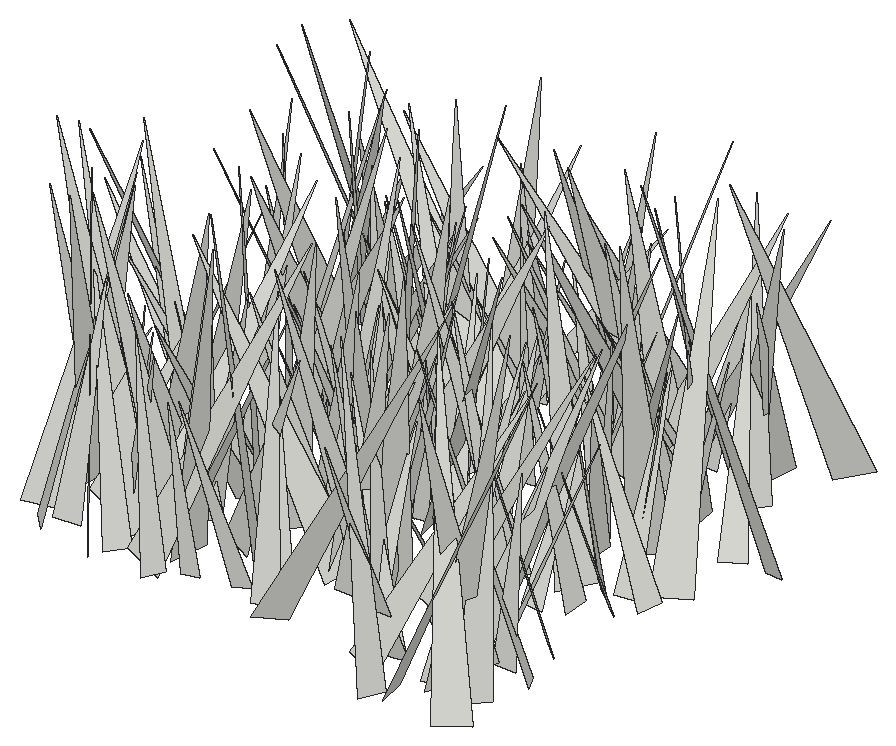
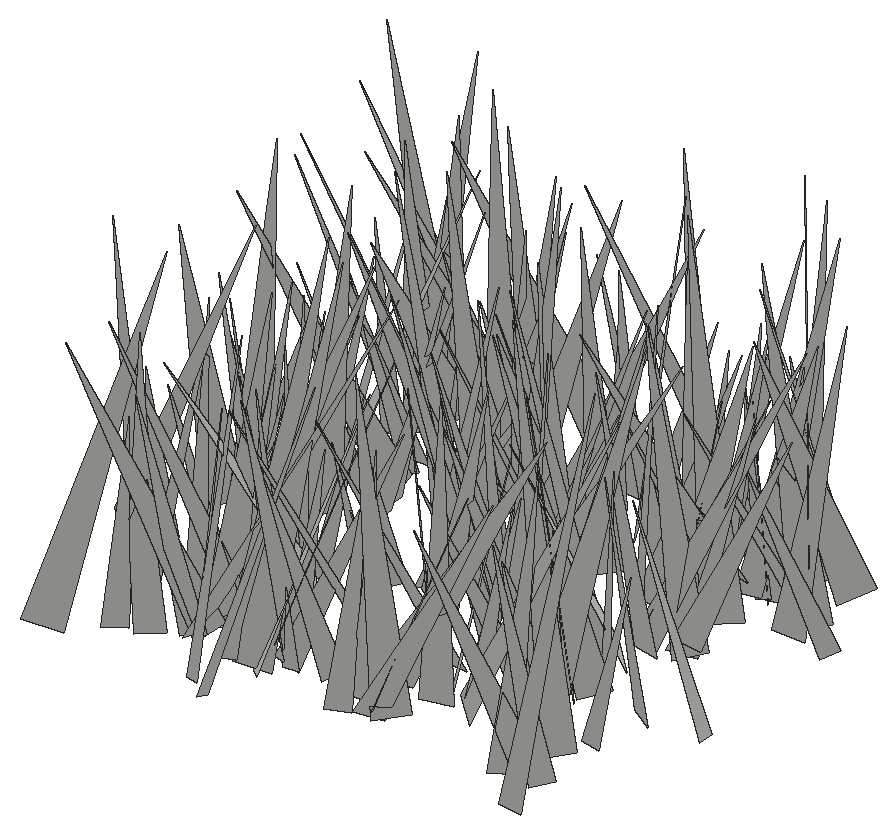
# SketchUp Ruby script. Lengths in inches.
U = 1.inch
M = Sketchup.active_model
def pt(a) = Geom::Point3d.new(a.map { |v| v * U })
def face(e, loops, mat)
  f = e.add_face(loops[0].map { |a| pt(a) })
  loops[1..].each { |l| e.add_face(l.map { |a| pt(a) }).erase! }
  f.material = f.back_material = mat if mat
  f
end
# faces: each face lists its corners as indices into pts; further lists are holes
def faces(e, pts, list, mat = nil) = list.each { |f| face(e, (f[0].is_a?(Array) ? f : [f]).map { |l| l.map { |i| pts[i] } }, mat) }
# xy, xz, yz: faces in a plane at the given z, y or x. An outline is a flat list of corners, or four numbers for a rectangle; further outlines are holes
def ring(l) = l.size == 4 ? [[l[0], l[1]], [l[2], l[1]], [l[2], l[3]], [l[0], l[3]]] : l.each_slice(2).to_a
def flat(e, list, mat, &to3) = list.each { |f| face(e, (f[0].is_a?(Array) ? f : [f]).map { |l| ring(l).map { |u, v| to3.(u, v) } }, mat) }
def xy(e, z, list, mat = nil) = flat(e, list, mat) { |x, y| [x, y, z] }
def xz(e, y, list, mat = nil) = flat(e, list, mat) { |x, z| [x, y, z] }
def yz(e, x, list, mat = nil) = flat(e, list, mat) { |y, z| [x, y, z] }
def lines(e, pts, list) = list.each { |a, b| e.add_line(pt(pts[a]), pt(pts[b])) }
# prism: a flat outline (further loops are holes) pulled along v
def prism(e, loops, v, mat = nil)
  f = face(e, loops, mat); d = Geom::Vector3d.new(v.map { |x| x * U })
  f.pushpull(f.normal.samedirection?(d) ? d.length : -d.length)
end
def box(e, o, s, mat = nil) = prism(e, [[o, [o[0] + s[0], o[1], o[2]], [o[0] + s[0], o[1] + s[1], o[2]], [o[0], o[1] + s[1], o[2]]]], [0, 0, s[2]], mat)
def at(x, y, z, deg = 0) = Geom::Transformation.translation(pt([x, y, z])) * Geom::Transformation.rotation(ORIGIN, Z_AXIS, deg.degrees)
def axes(o, x, y, z) = Geom::Transformation.new([*x, 0, *y, 0, *z, 0, *pt(o).to_a, 1])
def part(name) = M.definitions.add(name)
# library, detail: a bought-in or finely detailed component or shape, given as its bounding box
def library(name, o, s) = part(name).tap { |d| box(d.entities, o, s) }
def detail(e, o, s) = box(e.add_group.entities, o, s)
def put(e, d, t, mat = nil) = e.add_instance(d, t).tap { |i| i.material = mat if mat }
def group(e, t, mat = nil) = e.add_group.tap { |g| g.transformation = t; g.material = mat if mat }.entities
root = M.entities
c1 = part("fur_instance\#9")
p = [[0.8125,0,1.79],[0.67,-0.02,1.48],[0,-0.11,0],[0,0.11,0]]
faces(c1.entities,p,[[0,1,2,3]])
put(root,c1,axes([131.23,233.45,-27.1],[-0.49716,-5.04462,0.80589],[-5.07325,0.39247,-0.67299],[-0.59982,0.86174,5.02418]))
put(root,c1,axes([132.2,230.66,-27.1],[-6.81045,0.95525,0.6863],[0.79996,6.71798,-1.4123],[0.86231,1.31226,6.73054]))
put(root,c1,axes([134.09,234.68,-27.1],[5.76412,-4.56343,1.38579],[-4.26746,-5.90574,-1.69745],[-2.12934,-0.51736,7.15322]))
put(root,c1,axes([135.99,230.72,-27.1],[-2.86004,7.00076,0.77945],[7.00763,2.7424,1.08181],[-0.71502,-1.12544,7.48466]))
put(root,c1,axes([132.64,231.29,-27.1],[7.12948,2.21776,0.41944],[2.17259,-7.11974,0.71624],[-0.61174,0.56098,7.43203]))
put(root,c1,axes([133.92,232.91,-27.1],[7.67247,-2.21843,2.0813],[-2.41925,-7.8734,0.52613],[-1.84403,1.09916,7.96941]))
put(root,c1,axes([116.74,233.03,-27.1],[-5.8561,-4.67693,3.47291],[-5.12361,6.47844,0.0849],[2.77191,2.09401,7.49403]))
put(root,c1,axes([120.1,232.73,-27.1],[-4.33048,1.8912,1.2808],[1.94847,4.49129,-0.04381],[1.19187,-0.47097,4.72523]))
put(root,c1,axes([123.3,234.03,-27.1],[0.25989,-4.12749,1.06746],[-4.12688,-0.51192,-0.97467],[-1.06982,0.97209,4.01917]))
put(root,c1,axes([121.22,233.55,-27.1],[0.17752,-3.57602,1.3313],[-3.7929,-0.31113,-0.32997],[-0.41733,1.30655,3.56518]))
put(root,c1,axes([120.11,234.85,-27.1],[7.47084,-2.00529,1.5784],[-1.88161,-7.62701,-0.78379],[-1.72397,-0.36551,7.69548]))
put(root,c1,axes([130.46,232.25,-27.1],[1.42855,6.69806,0.59183],[6.31436,-1.12829,-2.47201],[2.31152,-1.05735,6.38701]))
put(root,c1,axes([125.57,232.85,-27.1],[7.23014,-2.66142,0.8801],[-2.79977,-6.73645,2.62947],[0.1379,2.76941,7.24182]))
put(root,c1,axes([130.05,233.93,-27.1],[-5.84783,-0.54956,0.92386],[-0.66437,5.86496,-0.71656],[0.84507,0.80798,5.82972]))
put(root,c1,axes([135.58,232.58,-27.1],[-6.65914,2.85732,1.17721],[2.6023,6.69305,-1.52492],[1.66678,0.96593,7.084]))
put(root,c1,axes([115.02,233.91,-27.1],[-0.99114,4.85366,1.48422],[5.00835,1.18049,-0.51592],[0.82303,-1.33855,4.92689]))
put(root,c1,axes([119.22,233.21,-27.1],[1.74287,7.71217,1.36191],[7.45298,-1.20484,-2.71503],[2.4053,-1.85492,7.42588]))
put(root,c1,axes([119.18,235.42,-27.1],[-7.26017,0.65472,1.63239],[0.85,7.37598,0.82207],[1.53976,-0.9847,7.24313]))
put(root,c1,axes([113.81,237.31,-27.1],[7.57168,-2.77915,1.4038],[-2.39268,-7.55557,-2.05259],[-1.99233,-1.48808,7.80006]))
put(root,c1,axes([117.86,233.37,-27.1],[-5.44212,1.96061,0.21811],[1.90755,5.39324,-0.88463],[0.50284,0.7598,5.71648]))
put(root,c1,axes([130.01,234.07,-27.1],[-5.54219,0.95074,1.40051],[0.80502,5.69802,-0.68242],[1.48905,0.4581,5.58158]))
put(root,c1,axes([124.8125,233.51,-27.1],[-0.46142,6.00885,1.03301],[6.04976,0.32253,0.82618],[-0.75742,-1.08443,5.96964]))
put(root,c1,axes([136.26,235.08,-27.1],[-5.87124,-3.56524,0.53214],[-3.58838,5.68376,-1.51131],[-0.34307,1.5651,6.70063]))
put(root,c1,axes([130.94,233.49,-27.1],[-1.18961,5.30841,0.21099],[4.92708,1.02155,2.07828],[-1.98686,-0.64508,5.02744]))
put(root,c1,axes([127,236.125,-27.1],[2.07554,-6.96607,1.71735],[-7.11885,-1.77704,1.39545],[0.89291,2.02467,7.13349]))
put(root,c1,axes([122.99,235.46,-27.1],[-6.35073,-3.49942,2.22612],[-3.7296,6.59945,-0.26567],[1.81428,1.31702,7.24617]))
put(root,c1,axes([134.78,235.35,-27.1],[-0.53957,3.97433,2.02364],[4.38519,0.84425,-0.48882],[0.81275,-1.91664,3.98089]))
put(root,c1,axes([114.22,233.26,-27.1],[5.15399,5.0376,1.12923],[4.93282,-5.27609,1.02292],[-1.5231,-0.04087,7.13405]))
put(root,c1,axes([124.59,234.8,-27.1],[-2.6188,2.85202,1.01974],[2.95253,2.70449,0.01846],[0.67563,-0.76402,3.87193]))
put(root,c1,axes([129.3,234.06,-27.1],[-2.23012,3.65012,0.738],[3.54975,2.34365,-0.86487],[1.12574,-0.15918,4.18913]))
put(root,c1,axes([116.7,235.36,-27.1],[2.33806,3.32528,1.40975],[3.5899,-2.32407,-0.47188],[-0.3968,-1.43269,4.03749]))
put(root,c1,axes([121.08,236.46,-27.1],[-0.06945,-5.66946,1.63507],[-5.27402,0.7929,2.5253],[2.64594,1.43164,5.07647]))
put(root,c1,axes([116.05,236.6,-27.1],[-0.58442,-4.16845,1.10453],[-3.96593,0.95723,1.51414],[1.69333,0.80327,3.92746]))
put(root,c1,axes([127.69,236.53,-27.1],[-1.28539,6.13898,3.44989],[6.89976,0.39684,1.86462],[-1.40785,-3.66012,5.98853]))
put(root,c1,axes([127.63,237.45,-27.1],[3.37968,-7.43588,1.46776],[-7.57694,-3.27406,0.85991],[0.19143,1.6903,8.12251]))
put(root,c1,axes([125.64,237.22,-27.1],[-6.93796,2.79801,1.11968],[3.01121,6.55067,2.28891],[0.12298,-2.54512,7.12215]))
put(root,c1,axes([116.3,236.6,-27.1],[-4.3642,6.37446,3.0679],[7.06974,4.05938,1.62241],[0.25406,-3.46117,7.553]))
put(root,c1,axes([135.3,237.49,-27.1],[-3.21192,-3.98216,0.77509],[-3.98629,3.28152,0.34045],[0.75355,0.38579,5.10471]))
put(root,c1,axes([133.55,232.78,-27.1],[-6.0414,2.82747,0.77084],[2.14541,5.47009,-3.25002],[1.99649,2.67784,5.82499]))
put(root,c1,axes([115.99,236.46,-27.1],[3.13173,2.6382,1.54856],[2.8558,-3.31576,-0.12654],[-1.0966,-1.10068,4.0929]))
put(root,c1,axes([113.33,237.09,-27.1],[4.2743,-5.66959,1.70794],[-5.91958,-4.14155,1.06631],[-0.14077,2.00854,7.01974]))
put(root,c1,axes([117.75,238.3,-27.1],[3.73697,-5.4189,0.58942],[-5.45085,-3.71358,0.41766],[0.01126,0.72231,6.56925]))
put(root,c1,axes([116.83,238.96,-27.1],[4.42124,-3.27,0.9733],[-2.9097,-4.44582,-1.71927],[-1.78153,-0.85401,5.22344]))
put(root,c1,axes([117.72,234.78,-27.1],[-0.98442,7.82804,0.7856],[7.24103,0.59195,3.17514],[-3.07617,-1.11168,7.22258]))
put(root,c1,axes([130.6,236.27,-27.1],[4.59981,5.90875,0.46757],[5.722,-4.27232,-2.30133],[1.54616,-1.76752,7.12569]))
put(root,c1,axes([113.44,234.3,-27.1],[-5.30404,4.85737,1.41696],[4.30663,5.41145,-2.42976],[2.65607,0.92563,6.76928]))
put(root,c1,axes([113.57,238.22,-27.1],[0.65749,-6.30029,1.7132],[-6.47052,-0.85883,-0.67511],[-0.87239,1.62165,6.29842]))
put(root,c1,axes([124.79,236.92,-27.1],[2.82445,3.52777,0.66946],[3.53756,-2.58781,-1.2883],[0.61561,-1.31488,4.33162]))
put(root,c1,axes([116.1,238.99,-27.1],[3.30529,-7.09092,0.75642],[-7.06387,-3.14139,1.41833],[0.97724,1.27626,7.69379]))
put(root,c1,axes([119.27,239.47,-27.1],[0.9036,-5.03288,0.01557],[-4.93923,-0.88981,-0.97923],[-0.96652,-0.158,5.01871]))
put(root,c1,axes([124.92,237.94,-27.1],[-5.6933,-0.47947,0.5538],[-0.44449,5.71072,0.37467],[0.58224,-0.32872,5.70116]))
put(root,c1,axes([118.86,237.61,-27.1],[4.80209,-1.99507,1.20954],[-2.10711,-4.89697,0.2883],[-1.00169,0.73669,5.19204]))
put(root,c1,axes([132.38,237.31,-27.1],[0.51441,-3.71167,1.78135],[-3.92489,0.09986,1.3415],[1.24297,1.85145,3.49879]))
put(root,c1,axes([132.69,236.44,-27.1],[2.40606,6.39383,1.08481],[6.38564,-2.13376,-1.58675],[1.13207,-1.55339,6.64473]))
put(root,c1,axes([114.79,236.07,-27.1],[1.15422,4.7345,0.08294],[4.6056,-1.10261,-1.15208],[1.10037,-0.35121,4.73502]))
put(root,c1,axes([118.68,236.52,-27.1],[4.79219,0.94532,0.41054],[0.81575,-4.67249,1.23678],[-0.62985,1.14081,4.72537]))
put(root,c1,axes([128.04,236.54,-27.1],[5.65388,1.0827,1.74004],[0.6959,-5.81697,1.3583],[-1.92762,1.07564,5.59407]))
put(root,c1,axes([121.86,238.68,-27.1],[5.17414,-4.36417,1.70527],[-4.54977,-5.28673,0.27499],[-1.1196,1.31532,6.76329]))
put(root,c1,axes([127.16,237.09,-27.1],[-1.66344,3.87519,0.54462],[3.91265,1.65754,0.1564],[0.06977,-0.56232,4.21422]))
put(root,c1,axes([129.25,238.89,-27.1],[-2.36065,-3.34559,0.0438],[-3.13879,2.19578,-1.44709],[-1.15883,0.86782,3.83035]))
put(root,c1,axes([111.43,238.36,-27.1],[2.74116,-2.85153,0.16279],[-2.64199,-2.44575,1.64616],[1.08517,1.2485,3.59657]))
put(root,c1,axes([117.92,239.28,-27.1],[-3.40624,-2.616,1.08161],[-2.59295,3.56228,0.44999],[1.13575,0.28715,4.27123]))
put(root,c1,axes([129.46,237.39,-27.1],[0.97735,4.73028,0.44464],[4.65378,-0.86171,-1.06216],[0.95682,-0.64061,4.71196]))
put(root,c1,axes([132.86,238.52,-27.1],[4.03846,2.29721,0.25382],[2.30928,-3.98992,-0.63131],[0.09403,-0.6739,4.60302]))
put(root,c1,axes([119.08,237.21,-27.1],[-0.71343,7.62578,1.29035],[7.14993,0.15622,3.02994],[-2.94889,-1.46615,7.03427]))
put(root,c1,axes([118.04,241.1,-27.1],[-5.4355,-1.48683,0.1699],[-1.41481,5.31415,1.24191],[0.48767,-1.15472,5.49664]))
put(root,c1,axes([129.49,239.09,-27.1],[-4.34694,-0.07841,1.0456],[-0.20123,4.43859,-0.5037],[1.02905,0.53671,4.31837]))
put(root,c1,axes([124.08,241.12,-27.1],[-1.04012,-7.65192,1.88155],[-7.84849,1.17518,0.4406],[0.70237,1.80029,7.70971]))
put(root,c1,axes([117.26,236.75,-27.1],[-0.93463,7.10607,0.24964],[6.82555,0.96718,-1.97702],[1.99262,0.02006,6.88921]))
put(root,c1,axes([123.86,240.25,-27.1],[-2.53875,-3.10556,0.31926],[-3.0835,2.42999,-0.88252],[-0.48832,0.80145,3.91291]))
put(root,c1,axes([121.82,241.17,-27.1],[2.30675,-6.01681,0.97122],[-6.03702,-2.11321,1.24701],[0.83643,1.34116,6.32203]))
put(root,c1,axes([125.18,238.93,-27.1],[4.28943,0.41298,0.87796],[0.18379,-4.25331,1.1028],[-0.95267,1.03894,4.16576]))
put(root,c1,axes([133.97,240.64,-27.1],[-5.16901,0.01394,1.37798],[0.15537,5.32107,0.52899],[1.36927,-0.55116,5.14189]))
put(root,c1,axes([117.46,238.6875,-27.1],[-6.47288,0.26814,0.01301],[0.25719,6.28405,-1.55397],[0.07694,1.55212,6.2893]))
put(root,c1,axes([131.41,239.67,-27.1],[-5.82181,0.2065,0.70872],[0.14567,5.84473,-0.50632],[0.72368,0.48471,5.80343]))
put(root,c1,axes([123.96,238.7,-27.1],[4.21835,1.12148,1.8478],[0.48542,-4.44001,1.58659],[-2.10629,1.22277,4.06632]))
put(root,c1,axes([131.12,240.8,-27.1],[-7.49054,-0.65717,0.9559],[-0.61994,7.54719,0.33069],[0.98046,-0.24861,7.51203]))
put(root,c1,axes([118.9375,240.48,-27.1],[-4.32305,-4.69404,2.5219],[-5.10648,4.57733,-0.23372],[1.52244,2.02405,6.37716]))
put(root,c1,axes([117.51,241.85,-27.1],[-3.5976,-6.50533,0.64098],[-6.34012,3.29439,-2.15004],[-1.59153,1.58132,7.11613]))
put(root,c1,axes([126.53,241.64,-27.1],[2.79226,2.81825,2.22878],[3.51982,-2.71249,-0.9798],[-0.72174,-2.32521,3.84438]))
put(root,c1,axes([125.8,242.45,-27.1],[7.87771,-0.03675,0.30438],[0.03502,-7.66773,-1.83222],[-0.30459,-1.83219,7.66177]))
put(root,c1,axes([135.26,241.18,-27.1],[-2.96371,-3.18096,0.56073],[-3.21747,2.84043,-0.89238],[-0.28422,1.01488,4.25508]))
put(root,c1,axes([123.08,239.76,-27.1],[2.64419,5.03318,0.33977],[4.95036,-2.51506,-1.26831],[0.97076,-0.88412,5.54221]))
put(root,c1,axes([115.47,241.7,-27.1],[5.59181,-3.37862,1.09906],[-3.46581,-5.63815,0.30113],[-0.78177,0.82912,6.52631]))
put(root,c1,axes([132.68,239.64,-27.1],[-0.04754,4.40868,0.34675],[4.41199,0.07095,-0.29716],[0.30179,-0.34273,4.39891]))
put(root,c1,axes([124.6,242.14,-27.1],[3.42079,-7.2545,1.9343],[-7.49487,-3.17419,1.34998],[0.44283,2.31686,7.90614]))
put(root,c1,axes([131.85,238.61,-27.1],[7.63616,1.08232,1.22596],[0.61242,-7.3209,2.64853],[-1.51635,2.49367,7.24345]))
put(root,c1,axes([115.83,241.76,-27.1],[-4.20776,3.77593,1.0344],[3.85861,3.7428,2.0336],[-0.66241,-2.18328,5.27517]))
put(root,c1,axes([124.6875,241.78,-27.1],[2.97768,-2.23657,0.59018],[-2.29034,-2.98547,0.24174],[-0.32391,0.5494,3.71623]))
put(root,c1,axes([122.9,239.47,-27.1],[-3.04551,1.64304,1.0176],[0.80196,2.80235,-2.12461],[1.7584,1.56764,2.73144]))
put(root,c1,axes([134.17,242.07,-27.1],[-2.56443,-3.19615,1.19823],[-3.34404,2.653,-0.08027],[0.6845,0.98675,4.09698]))
put(root,c1,axes([124.12,238.28,-27.1],[-7.01528,2.7432,0.95764],[2.14491,6.5776,-3.12905],[1.96,2.6204,6.85188]))
put(root,c1,axes([122.43,242.78,-27.1],[-0.63614,-4.28295,0.71253],[-4.25699,0.4736,-0.95381],[-0.85404,0.8295,4.22357]))
put(root,c1,axes([133.02,241.85,-27.1],[-6.40886,3.74132,2.19702],[3.96061,6.64492,0.23769],[1.77143,-1.32114,7.41717]))
put(root,c1,axes([136.16,242.34,-27.1],[-4.59292,1.38597,0.57425],[1.45174,4.5724,0.57548],[0.37836,-0.71958,4.76284]))
put(root,c1,axes([128.11,240.36,-27.1],[-0.8094,5.47668,0.09308],[5.43232,0.79056,0.72297],[-0.70181,-0.19701,5.48875]))
put(root,c1,axes([122.48,243.19,-27.1],[-4.6508,-5.63712,0.37429],[-5.36466,4.25457,-2.58191],[-1.77136,1.91537,6.83673]))
put(root,c1,axes([122.11,242.9375,-27.1],[-1.05055,-3.99645,1.56356],[-4.12582,0.49771,-1.49997],[-1.18067,1.81677,3.85037]))
put(root,c1,axes([123.86,242.57,-27.1],[0.25719,7.17904,2.90731],[6.91163,1.10018,-3.3281],[3.49578,-2.70337,6.36621]))
put(root,c1,axes([126.64,243.67,-27.1],[-5.33847,-0.05884,0.40473],[-0.0096,5.31499,0.64603],[0.40887,-0.64342,5.29956]))
put(root,c1,axes([132.07,244.41,-27.1],[4.60045,-1.39498,0.802],[-1.20201,-4.59424,-1.0961],[-1.06973,-0.83684,4.68067]))
put(root,c1,axes([116.97,242.47,-27.1],[1.78136,5.8506,1.71123],[6.09225,-1.76893,-0.29408],[-0.20572,-1.72409,6.10871]))
put(root,c1,axes([125.85,244.33,-27.1],[-3.47477,-5.64058,1.59223],[-5.83486,3.50381,-0.32112],[0.55295,1.52727,6.61718]))
put(root,c1,axes([135,242.38,-27.1],[-1.136,4.49998,0.83575],[4.53043,1.22799,-0.4539],[0.65076,-0.69355,4.61891]))
put(root,c1,axes([133.57,245.58,-27.1],[4.47344,-6.57845,1.38646],[-6.62258,-4.59864,-0.45163],[-1.15746,0.88686,7.94253]))
put(root,c1,axes([134.4,243.65,-27.1],[4.12014,1.91723,1.34742],[2.03951,-4.27599,-0.15214],[-1.154,-0.71202,4.54182]))
put(root,c1,axes([117.89,243.93,-27.1],[2.9133,6.77269,2.26525],[7.08174,-2.424,-1.8604],[0.9217,-2.7826,7.13411]))
put(root,c1,axes([117.75,247.2,-27.1],[5.40513,-4.44008,1.03103],[-3.91993,-5.34397,-2.46351],[-2.32626,-1.31164,6.54682]))
put(root,c1,axes([123.17,243.36,-27.1],[-6.34859,-2.07949,3.15929],[-2.7531,6.77324,-1.07409],[2.59343,2.09974,6.59357]))
put(root,c1,axes([122.86,243.125,-27.1],[5.61181,2.09612,1.30854],[1.89864,-5.73587,1.04566],[-1.58152,0.55181,5.89854]))
put(root,c1,axes([124.49,242.6875,-27.1],[2.31766,5.02687,0.82298],[4.84651,-2.45447,1.34356],[-1.56781,-0.15629,5.3699]))
put(root,c1,axes([122.39,243.47,-27.1],[-5.96382,1.04535,0.88629],[0.82737,5.90096,-1.39268],[1.09259,1.23747,5.8924]))
put(root,c1,axes([127.43,244.27,-27.1],[-2.50227,2.59124,1.1484],[2.47228,2.74461,-0.80603],[1.38608,-0.21748,3.51087]))
put(root,c1,axes([116.39,246.23,-27.1],[2.55754,-6.5759,0.86107],[-6.14173,-2.00015,2.96707],[2.50263,1.81158,6.40156]))
put(root,c1,axes([131.16,245.77,-27.1],[-1.15878,-4.12917,1.68532],[-4.31214,1.48176,0.66553],[1.13832,1.40977,4.23673]))
put(root,c1,axes([130.01,245.74,-27.1],[-1.05409,-4.02831,1.60299],[-4.27873,0.70037,-1.05356],[-0.69957,1.78611,4.02845]))
put(root,c1,axes([136.31,243.4375,-27.1],[-5.32969,5.59283,1.04722],[5.46672,5.43108,-1.18331],[1.57839,0.07463,7.63447]))
put(root,c1,axes([111.1,246.22,-27.1],[4.64757,1.11707,0.03174],[1.0994,-4.54603,-0.98676],[0.20042,-0.96672,4.67697]))
put(root,c1,axes([124.5,245.95,-27.1],[3.53151,3.08583,1.68165],[3.37882,-3.63698,-0.42174],[-0.96639,-1.43941,4.67077]))
put(root,c1,axes([117.125,244.68,-27.1],[2.66286,4.62658,1.9724],[4.32664,-3.24515,1.77077],[-2.56433,-0.67099,5.03592]))
put(root,c1,axes([119.32,246.72,-27.1],[3.99412,4.65299,3.2629],[5.30006,-4.48907,-0.08624],[-2.05092,-2.53923,6.13155]))
put(root,c1,axes([116.52,249.39,-27.1],[4.04445,-6.42376,0.8146],[-6.13253,-4.10829,-1.94934],[-2.07854,-0.37835,7.33638]))
put(root,c1,axes([122.39,245.03,-27.1],[7.1658,2.76652,1.69463],[2.58302,-7.35112,1.0785],[-1.96302,0.42601,7.60521]))
put(root,c1,axes([117.43,243.28,-27.1],[4.44404,5.53922,0.27989],[5.13876,-4.2472,2.46279],[-2.08674,1.3376,6.66087]))
put(root,c1,axes([120.92,247.37,-27.1],[1.65267,-3.08975,1.39314],[-3.11179,-1.99748,-0.7386],[-1.34319,0.82596,3.42525]))
put(root,c1,axes([130.18,248.58,-27.1],[6.41369,-0.07562,0.05633],[-0.05586,-6.13403,-1.87481],[-0.07597,-1.87412,6.13403]))
put(root,c1,axes([133.49,248.71,-27.1],[5.23051,-1.10724,0.78196],[-0.81536,-5.06,-1.7109],[-1.08287,-1.53819,5.06527]))
put(root,c1,axes([138.26,247.12,-27.1],[-4.4516,-6.59475,1.62319],[-6.65602,3.85048,-2.61027],[-1.35017,2.76139,7.51625]))
put(root,c1,axes([133.38,245.99,-27.1],[-5.0928,-0.09663,0.30052],[-0.16718,4.94609,-1.24277],[0.26777,1.25023,4.93978]))
put(root,c1,axes([117.98,247.31,-27.1],[4.10331,-3.61689,0.17449],[-3.47529,-3.85943,1.7253],[1.0172,1.40442,5.19061]))
put(root,c1,axes([124.27,245.75,-27.1],[-6.63605,2.7216,0.19643],[2.70208,6.62626,-0.52374],[0.38006,0.41041,7.15332]))
put(root,c1,axes([134.29,246.53,-27.1],[3.78689,-0.0231,1.24793],[-0.32688,-3.86581,0.92039],[-1.20458,0.97644,3.67342]))
put(root,c1,axes([130.89,250.36,-27.1],[0.06912,-7.57158,0.2529],[-7.42195,-0.11839,-1.51598],[-1.51902,0.23392,7.41859]))
put(root,c1,axes([113.92,246.57,-27.1],[2.58353,5.00263,1.49189],[5.09313,-2.78069,0.50442],[-1.14546,-1.08079,5.60772]))
put(root,c1,axes([130.99,249.43,-27.1],[5.55902,-2.83125,1.90418],[-2.404,-5.83322,-1.65498],[-2.42129,-0.70867,6.01496]))
put(root,c1,axes([117.3,246.45,-27.1],[4.85297,5.01471,2.08252],[4.89411,-5.24941,1.23566],[-2.35199,-0.5761,6.86817]))
put(root,c1,axes([126.67,246.875,-27.1],[1.26657,4.59176,1.22685],[4.36989,-1.62436,1.56816],[-1.86909,-0.68616,4.4977]))
put(root,c1,axes([116.08,248.87,-27.1],[0.58274,-3.68979,0.92218],[-3.78198,-0.46356,0.53511],[0.40205,0.98748,3.697]))
put(root,c1,axes([124.22,248.38,-27.1],[2.61371,2.45973,0.53308],[2.49517,-2.43181,-1.01309],[0.32949,-1.09634,3.44317]))
put(root,c1,axes([134.39,250.3,-27.1],[-1.58112,-4.73276,0.31075],[-4.65779,1.61119,0.83937],[0.89473,0.02406,4.91878]))
put(root,c1,axes([120.67,249.43,-27.1],[-3.88391,-3.01754,1.00768],[-2.99103,4.00531,0.46572],[1.08383,0.24005,4.89626]))
put(root,c1,axes([114.58,250.64,-27.1],[8.18505,-1.50624,0.16494],[-1.43272,-7.98824,-1.85106],[-0.49323,-1.79175,8.11402]))
put(root,c1,axes([125.53,247.875,-27.1],[4.20313,-0.16718,1.34956],[-0.39887,-4.34286,0.70427],[-1.30006,0.79192,4.14708]))
put(root,c1,axes([136.42,246.95,-27.1],[-3.1637,4.01487,0.30871],[3.99884,3.17867,-0.35895],[0.47305,-0.01931,5.09895]))
put(root,c1,axes([128.39,250.22,-27.1],[-5.1626,-2.88411,0.4563],[-2.82641,5.16852,0.6903],[0.7333,-0.3834,5.87316]))
put(root,c1,axes([130.2,250.78,-27.1],[2.51881,-4.55482,0.15905],[-4.51842,-2.51942,-0.59372],[-0.59628,-0.14918,5.17091]))
put(root,c1,axes([118.09,248.03,-27.1],[4.70172,-1.10111,0.26171],[-1.12934,-4.49092,1.39405],[0.07438,1.41645,4.62334]))
put(root,c1,axes([114.15,249.32,-27.1],[-0.09942,-3.58739,1.13729],[-3.70553,-0.10534,-0.65623],[-0.65715,1.13676,3.52826]))
put(root,c1,axes([131.42,251.23,-27.1],[-3.70308,-3.24105,0.05421],[-3.08159,3.54543,1.46762],[1.00557,-1.07036,4.69716]))
put(root,c1,axes([128.72,248.48,-27.1],[-0.54656,4.2534,1.19948],[4.32093,0.26075,1.04426],[-0.92722,-1.29209,4.15928]))
put(root,c1,axes([130.02,249.33,-27.1],[-3.10303,1.40825,1.48641],[1.65077,3.31728,0.3033],[1.21143,-0.91317,3.39411]))
put(root,c1,axes([119.58,249.4,-27.1],[-3.58724,1.8714,1.40372],[2.1412,3.66165,0.59026],[0.94225,-1.19623,4.00275]))
put(root,c1,axes([128.3,252.38,-27.1],[6.29678,-5.28708,1.00032],[-4.88133,-6.26054,-2.36253],[-2.26416,-1.20654,7.87535]))
put(root,c1,axes([119.46,250.14,-27.1],[-4.9129,-5.75828,0.52895],[-5.68371,4.68095,-1.83254],[-1.06438,1.58274,7.34412]))
put(root,c1,axes([131,251.9,-27.1],[-8.10416,-1.22815,0.06312],[-1.16757,7.81624,2.17553],[0.38615,-2.14192,7.90272]))
put(root,c1,axes([127.72,252.54,-27.1],[0.59961,-8.00132,0.48644],[-8.01433,-0.60861,-0.13198],[-0.1682,0.47514,8.02267]))
put(root,c1,axes([126.86,251.57,-27.1],[0.11807,-5.18176,0.38422],[-4.95689,-0.22756,-1.54584],[-1.55804,0.33133,4.94722]))
put(root,c1,axes([117.26,248.94,-27.1],[-0.85461,3.70026,0.75554],[3.7566,0.91253,-0.21994],[0.38824,-0.68446,3.79129]))
put(root,c1,axes([130.57,250.87,-27.1],[4.49335,-4.83843,2.48866],[-4.8443,-5.0271,-1.02712],[-2.47721,1.05444,6.5227]))
put(root,c1,axes([121.8,247.8,-27.1],[1.69788,6.23349,0.03172],[6.16311,-1.67374,-0.97718],[0.93461,-0.28707,6.38626]))
put(root,c1,axes([128.71,249.63,-27.1],[0.78552,4.64999,1.51438],[4.88897,-0.70993,-0.35606],[0.11721,-1.55126,4.70241]))
put(root,c1,axes([127.33,252.87,-27.1],[-4.17954,-4.03403,0.06779],[-3.83281,4.00041,1.74723],[1.26,-1.21235,5.53978]))
put(root,c1,axes([129.81,246.15,-27.1],[5.70548,5.18554,0.14342],[4.71826,-5.27598,3.06024],[-2.15603,2.1765,7.07653]))
put(root,c1,axes([120.68,250.36,-27.1],[-1.61639,5.70202,2.80279],[6.31476,1.76115,0.05886],[0.70173,-2.71416,5.92641]))
put(root,c1,axes([122.23,252.13,-27.1],[-4.07436,-2.22938,0.28557],[-2.14023,4.02883,0.91657],[0.68639,-0.67121,4.55307]))
put(root,c1,axes([132.32,252.9,-27.1],[0.1957,-7.90399,1.09327],[-7.43409,0.21668,2.89722],[2.89871,1.0893,7.35646]))
put(root,c1,axes([123.125,250.05,-27.1],[-5.23637,6.32875,0.17784],[5.87309,4.76933,3.20385],[-2.36465,-2.16904,7.5636]))
put(root,c1,axes([123.1875,249.85,-27.1],[2.725,5.40327,0.30402],[4.86473,-2.29653,-2.78814],[2.3711,-1.498,5.37096]))
put(root,c1,axes([126.53,251.75,-27.1],[-1.2496,-4.95098,2.04852],[-4.91628,1.89585,1.58307],[2.13046,1.47094,4.85465]))
put(root,c1,axes([115.35,253.05,-27.1],[4.3108,-3.69492,0.61953],[-3.55093,-4.33068,-1.12044],[-1.19463,-0.46051,5.56597]))
put(root,c1,axes([129.79,250.11,-27.1],[0.86928,6.52033,1.58307],[6.24969,-0.2059,-2.58369],[2.44176,-1.79425,6.04937]))
put(root,c1,axes([133.65,253.37,-27.1],[4.86782,-2.47433,0.4659],[-2.27673,-4.75873,-1.48527],[-1.07512,-1.1257,5.25471]))
put(root,c1,axes([123.16,253.13,-27.1],[2.62732,-3.98087,0.28129],[-3.95197,-2.64215,-0.47983],[-0.55532,-0.03119,4.74551]))
put(root,c1,axes([134.47,250.7,-27.1],[-5.32179,3.05618,1.70346],[3.04909,5.5718,-0.47069],[1.71611,-0.42222,6.11884]))
put(root,c1,axes([113.47,254.98,-27.1],[-3.16063,-7.46069,0.64697],[-7.21635,3.22195,1.90087],[2.00118,-0.16476,7.87643]))
put(root,c1,axes([122.98,251.93,-27.1],[-0.34045,4.62028,2.07312],[5.05885,0.21591,0.34957],[-0.23002,-2.08976,4.6196]))
put(root,c1,axes([124.91,251.1875,-27.1],[3.82826,-1.89723,1.31218],[-2.241,-3.66166,1.2438],[-0.54703,1.72325,4.08754]))
put(root,c1,axes([113.6875,252.79,-27.1],[3.31192,-3.28223,0.0309],[-3.2384,-3.26025,0.79144],[0.53549,0.5836,4.59516]))
put(root,c1,axes([121.27,252.3,-27.1],[5.02607,-4.57327,2.19343],[-4.92834,-5.13329,0.59007],[-1.19892,1.92923,6.76964]))
put(root,c1,axes([130.97,252.03,-27.1],[1.98838,-4.24744,1.75797],[-4.57109,-1.62434,1.24561],[0.4862,2.09896,4.52138]))
put(root,c1,axes([128.9,254.71,-27.1],[-3.46675,-5.54657,1.13696],[-5.08588,3.63649,2.23277],[2.48816,-0.29493,6.14797]))
put(root,c1,axes([130.86,251.86,-27.1],[-4.62696,-2.40171,1.71965],[-2.7299,4.69747,-0.78458],[1.12828,1.51649,5.15378]))
put(root,c1,axes([121.99,252.74,-27.1],[-4.61226,3.61546,0.79034],[3.61757,4.1381,2.18138],[-0.78062,-2.18488,5.43931]))
put(root,c1,axes([126.95,250.69,-27.1],[-5.68198,1.58826,2.45655],[1.00817,6.10119,-1.61279],[2.74605,1.04639,5.67506]))
put(root,c1,axes([135.83,254.98,-27.1],[3.52912,-6.81057,1.30534],[-6.45742,-3.76145,-2.16695],[-2.52774,0.10047,7.35818]))
put(root,c1,axes([127.82,255.42,-27.1],[-5.63617,-2.55407,1.20627],[-1.85262,5.37498,2.72438],[2.13217,-2.08115,5.55585]))
put(root,c1,axes([130.61,251.46,-27.1],[6.21247,-1.9108,0.54363],[-1.98453,-5.88708,1.9863],[0.09123,2.05733,6.18874]))
put(root,c1,axes([114.43,252.51,-27.1],[3.95823,-3.37287,0.12226],[-3.1364,-3.60629,2.0534],[1.24667,1.63622,4.7778]))
